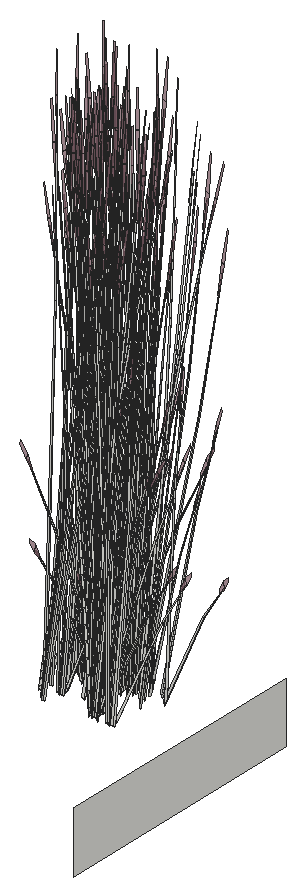
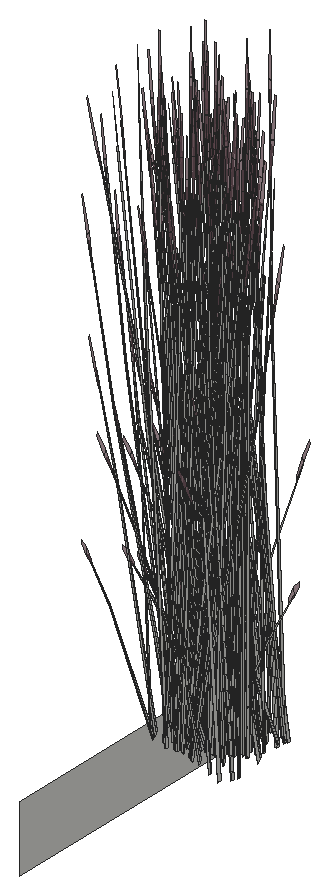
# SketchUp Ruby script. Lengths in inches.
U = 1.inch
M = Sketchup.active_model
def pt(a) = Geom::Point3d.new(a.map { |v| v * U })
def face(e, loops, mat)
  f = e.add_face(loops[0].map { |a| pt(a) })
  loops[1..].each { |l| e.add_face(l.map { |a| pt(a) }).erase! }
  f.material = f.back_material = mat if mat
  f
end
# faces: each face lists its corners as indices into pts; further lists are holes
def faces(e, pts, list, mat = nil) = list.each { |f| face(e, (f[0].is_a?(Array) ? f : [f]).map { |l| l.map { |i| pts[i] } }, mat) }
# xy, xz, yz: faces in a plane at the given z, y or x. An outline is a flat list of corners, or four numbers for a rectangle; further outlines are holes
def ring(l) = l.size == 4 ? [[l[0], l[1]], [l[2], l[1]], [l[2], l[3]], [l[0], l[3]]] : l.each_slice(2).to_a
def flat(e, list, mat, &to3) = list.each { |f| face(e, (f[0].is_a?(Array) ? f : [f]).map { |l| ring(l).map { |u, v| to3.(u, v) } }, mat) }
def xy(e, z, list, mat = nil) = flat(e, list, mat) { |x, y| [x, y, z] }
def xz(e, y, list, mat = nil) = flat(e, list, mat) { |x, z| [x, y, z] }
def yz(e, x, list, mat = nil) = flat(e, list, mat) { |y, z| [x, y, z] }
def lines(e, pts, list) = list.each { |a, b| e.add_line(pt(pts[a]), pt(pts[b])) }
# prism: a flat outline (further loops are holes) pulled along v
def prism(e, loops, v, mat = nil)
  f = face(e, loops, mat); d = Geom::Vector3d.new(v.map { |x| x * U })
  f.pushpull(f.normal.samedirection?(d) ? d.length : -d.length)
end
def box(e, o, s, mat = nil) = prism(e, [[o, [o[0] + s[0], o[1], o[2]], [o[0] + s[0], o[1] + s[1], o[2]], [o[0], o[1] + s[1], o[2]]]], [0, 0, s[2]], mat)
def at(x, y, z, deg = 0) = Geom::Transformation.translation(pt([x, y, z])) * Geom::Transformation.rotation(ORIGIN, Z_AXIS, deg.degrees)
def axes(o, x, y, z) = Geom::Transformation.new([*x, 0, *y, 0, *z, 0, *pt(o).to_a, 1])
def part(name) = M.definitions.add(name)
# library, detail: a bought-in or finely detailed component or shape, given as its bounding box
def library(name, o, s) = part(name).tap { |d| box(d.entities, o, s) }
def detail(e, o, s) = box(e.add_group.entities, o, s)
def put(e, d, t, mat = nil) = e.add_instance(d, t).tap { |i| i.material = mat if mat }
def group(e, t, mat = nil) = e.add_group.tap { |g| g.transformation = t; g.material = mat if mat }.entities
root = M.entities
M.materials.add("LightPink_Translucent").color = [144, 107, 117]
M.materials["LightPink_Translucent"].alpha = 0.75
c1 = part("blade")
p = [[2.15,0.21,22],[0,0.17,0],[0.09,0.45,0],[2.18,0.31,22],[2.29,0.31,22],[0.38,0.45,0],
  [2.48,0.24,33],[2.49,0.24,33],[2.48,0.22,33]]
faces(c1.entities,p,[[0,1,2,3],[4,5,2,3],[6,3,4,7],[8,0,3,6]])
c2 = part("seeds")
p = [[0.3,-0.1,1.38],[-0.01,-0.03,1.59],[-0.01,-0.03,0.03],[0.14,-0.07,-0.07],[0.29,-0.03,3],[0.15,0.01,3.11]]
faces(c2.entities,p,[[0,1,2,3],[1,0,4,5]],"LightPink_Translucent")
c3 = part("blade with seeds")
put(c3.entities,c1,at(0,0,0))
put(c3.entities,c2,axes([2.4,0.25,30.99],[1.5799,-0.05474,1.17369],[-0.12525,1.92788,0.29478],[-0.07173,-0.02425,1.56792]))
yz(root,346,[[14,42,40,48]])
put(root,c3,axes([334.63,24.32,49.95],[0.56491,0,0],[0,0.40454,0],[0,0,1.5764]))
put(root,c3,axes([339.08,29.64,49.82],[-0.52523,-0.06406,-0.55095],[0.11084,-0.39517,-0.1446],[-0.15674,-0.04788,1.21613]))
put(root,c3,axes([336.74,29.35,50.19],[0.47255,-0.19538,0.43871],[0.28245,0.35034,0],[-0.10763,0.0445,1.3917]))
put(root,c3,axes([334.83,24.28,50.3125],[0.47043,-0.11396,0.12794],[0.16474,0.32541,-0.36534],[0,0.07162,1.11991]))
put(root,c3,axes([335.26,27.95,50.09],[0.21952,0.43694,0.40429],[-0.62724,0.15194,0.15865],[0.00767,-0.08029,1.40366]))
put(root,c3,axes([335.16,27.9,49.95],[0.24498,-0.3521,-0.39531],[0.50902,0.16945,0.19025],[0,-0.08116,1.26923]))
put(root,c3,axes([335.79,29.03,49.95],[-0.16474,-0.33688,0],[0.47043,-0.11798,0],[0,0,1.36402]))
put(root,c3,axes([333.85,30.61,50.1],[-0.31568,-0.39156,0],[0.52815,-0.21836,-0.456],[0.12029,-0.04973,1.44655]))
put(root,c3,axes([334.67,24.3,50.36],[0.56863,0.18645,-0.25709],[-0.2738,0.39352,-0.44182],[0.01787,0.09662,1.41118]))
put(root,c3,axes([338.39,30.38,49.78],[-0.47255,-0.19538,-0.43871],[0.28245,-0.35034,0],[-0.10763,-0.0445,1.3917]))
put(root,c3,axes([338.18,27.47,49.32],[-0.04891,0.05148,1.55816],[-0.49427,0.11098,-0.23804],[-0.1194,-0.10096,0.26541]))
put(root,c3,axes([335.9,24.39,50.19],[0,-0.39075,0.43871],[0.56491,0,0],[0,0.089,1.3917]))
put(root,c3,axes([336.15,24.76,49.78],[0,0.39075,-0.43871],[-0.56491,0,0],[0,0.089,1.3917]))
put(root,c3,axes([337.42,28.15,50.1875],[-0.39671,-0.28463,0.15589],[0.39978,-0.27607,0.31002],[-0.04381,0.05813,1.41735]))
put(root,c3,axes([336.05,27.99,49.95],[0,-0.45213,0],[0.63136,0,0],[0,0,1.58567]))
put(root,c3,axes([335.46,28.07,50.15],[0.56891,0.18939,0.21263],[-0.2738,0.39352,0.44182],[0,-0.09071,1.41855]))
put(root,c3,axes([336.37,28.17,50.03],[0,0.45191,-0.04981],[-0.63136,0,0],[0,0.0142,1.58489]))
put(root,c3,axes([335.28,27.81,50.4],[-0.54829,0.02412,0.39531],[-0.04958,-0.40041,-0.19025],[0.09816,-0.04058,1.26923]))
put(root,c3,axes([338.1,24.99,50.29],[0.15933,-0.06164,1.26356],[0.39339,0.18587,-0.27174],[-0.11709,0.16083,0.54024]))
put(root,c3,axes([337.88,27.67,49.88],[-0.14565,0.31907,-0.0344],[-0.44829,-0.09815,-0.15595],[-0.06806,-0.05219,0.51438]))
put(root,c3,axes([335.02,27.12,50.1875],[-0.14586,0.38834,0.15589],[-0.53375,-0.1099,0.31002],[0.0922,-0.00189,1.41735]))
put(root,c3,axes([334.56,25.21,49.93],[0.53009,-0.13258,-0.16963],[0.18627,0.38191,0.00007],[0.05851,-0.01465,1.53656]))
put(root,c3,axes([338.55,27.27,50.29],[-0.03058,0.12783,1.26356],[-0.44698,0.10701,-0.27174],[-0.10448,-0.16522,0.54024]))
put(root,c3,axes([339.68,29.69,50.36],[-0.50979,0.25942,-0.25709],[-0.339,-0.36656,-0.44182],[-0.12578,-0.03723,1.41118]))
put(root,c3,axes([334.76,26.64,50.1],[-0.31568,-0.39156,0],[0.52815,-0.21836,-0.456],[0.12029,-0.04973,1.44655]))
put(root,c3,axes([334.57,24.08,49.95],[0.30332,0.32798,-0.39531],[-0.45944,0.23096,0.19025],[0.09816,0.04058,1.26923]))
put(root,c3,axes([336.64,27.14,50.1875],[-0.54257,0.10371,0.15589],[-0.13397,-0.38597,0.31002],[0.04839,0.05624,1.41735]))
put(root,c3,axes([337.64,29.13,50.1],[-0.63136,0,0],[0,-0.43672,-0.456],[0,-0.09947,1.44655]))
put(root,c3,axes([338.52,30.24,49.79],[-0.11861,-0.34048,-0.27372],[0.47106,-0.09668,0.27372],[-0.09497,-0.03926,1.22797]))
put(root,c3,axes([335.7,30.3,50.29],[-0.14352,0.07909,1.26356],[-0.42983,-0.13843,-0.27174],[0.07968,-0.17216,0.54024]))
put(root,c3,axes([335.75,27.7,50.09],[-0.41865,0.35461,0.40429],[-0.49737,-0.31303,0.15865],[0.10093,-0.03539,1.40366]))
put(root,c3,axes([334.42,25.45,50.29],[0.00891,-0.12953,1.26356],[0.4258,-0.14469,-0.27174],[0.13144,0.15503,0.54024]))
put(root,c3,axes([336.47,28.26,49.96],[0.35245,0.2524,0],[-0.35245,0.2524,0],[0,0,1.49564]))
put(root,c3,axes([336.46,27.97,50.4],[0.24498,-0.3521,0.39531],[0.50902,0.16945,-0.19025],[0,0.08116,1.26923]))
put(root,c3,axes([336.25,29.19,49.95],[0.50902,0.17543,0],[-0.24498,0.36452,0],[0,0,1.54589]))
put(root,c3,axes([340.02,23.79,49.82],[-0.34009,0.2937,-0.55095],[-0.42248,-0.26632,-0.1446],[-0.13628,0.07327,1.21613]))
put(root,c3,axes([334.28,30.55,49.78],[0.47255,-0.19538,-0.43871],[0.28245,0.35034,0],[0.10763,-0.0445,1.3917]))
put(root,c3,axes([338.125,29.01,50.06],[-0.46965,0.32852,0.27176],[-0.46994,-0.32506,-0.32244],[-0.0164,-0.09329,1.45692]))
put(root,c3,axes([336.3,27.88,50.1],[-0.63817,-0.08233,0.43472],[0.12987,-0.46497,0.17059],[0.09326,0.0449,1.50931]))
put(root,c3,axes([335.4,23.35,49.79],[0.11861,0.34048,-0.27372],[-0.47106,0.09668,0.27372],[0.09497,0.03926,1.22797]))
put(root,c3,axes([336.29,24.46,50.1],[0.63136,0,0],[0,0.43672,-0.456],[0,0.09947,1.44655]))
put(root,c3,axes([340.25,29.8125,50.18],[-0.49304,-0.31451,-0.2226],[0.41487,-0.35316,0.48713],[-0.13277,0.03679,1.48635]))
put(root,c3,axes([339.35,29.51,49.95],[-0.30332,-0.32798,-0.39531],[0.45944,-0.23096,0.19025],[-0.09816,-0.04058,1.26923]))
put(root,c3,axes([336.48,28.09,49.95],[0.56491,0,0],[0,0.40454,0],[0,0,1.5764]))
put(root,c3,axes([335.47,26.08,50.36],[-0.32378,-0.01225,0.92831],[0.21383,-0.26028,0.51254],[0.12791,0.09247,0.72818]))
put(root,c3,axes([335.93,27.64,50.4],[-0.30332,-0.32798,0.39531],[0.45944,-0.23096,-0.19025],[0.09816,0.04058,1.26923]))
put(root,c3,axes([335.38,27.72,50.36],[-0.05884,-0.44587,-0.25709],[0.6128,-0.02696,-0.44182],[0.10791,-0.05939,1.41118]))
put(root,c3,axes([336.67,28.05,50.3125],[0.47043,-0.11396,0.12794],[0.16474,0.32541,-0.36534],[0,0.07162,1.11991]))
put(root,c3,axes([338.95,30.42,50.19],[0.47255,0.19538,0.43871],[-0.28245,0.35034,0],[-0.10763,-0.0445,1.3917]))
put(root,c3,axes([335.3,26.74,49.79],[0.47106,0.09668,-0.27372],[-0.11861,0.34048,0.27372],[0.09497,-0.03926,1.22797]))
put(root,c3,axes([339.4,29.7,50.16],[0.13383,-0.46302,-0.20702],[0.63453,0.08071,0.45303],[-0.11087,-0.06394,1.38231]))
put(root,c3,axes([339.63,29.81,50.3125],[-0.09741,0.34873,0.12794],[-0.4759,-0.06053,-0.36534],[-0.08661,-0.03581,1.11991]))
put(root,c3,axes([337.75,28.17,50.19],[0,-0.39075,0.43871],[0.56491,0,0],[0,0.089,1.3917]))
put(root,c3,axes([335.19,26.58,49.78],[0.47255,-0.19538,-0.43871],[0.28245,0.35034,0],[0.10763,-0.0445,1.3917]))
put(root,c3,axes([340.58,24.59,49.78],[-0.47255,0.19538,-0.43871],[-0.28245,-0.35034,0],[-0.10763,0.0445,1.3917]))
put(root,c3,axes([334.84,31.35,49.82],[0.34009,-0.2937,-0.55095],[0.42248,0.26632,-0.1446],[0.13628,-0.07327,1.21613]))
put(root,c3,axes([337.78,28.83,49.78],[0,-0.39075,-0.43871],[0.56491,0,0],[0,-0.089,1.3917]))
put(root,c3,axes([338.02,29.2,50.19],[0,0.39075,0.43871],[-0.56491,0,0],[0,-0.089,1.3917]))
put(root,c3,axes([340.61,24.48,49.9375],[-0.31175,-0.39292,-0.04544],[0.52815,-0.21836,0.456],[-0.13015,0.03741,1.44584]))
put(root,c3,axes([336.14,27.55,50.3125],[0.09741,-0.34873,0.12794],[0.4759,0.06053,-0.36534],[0.08661,0.03581,1.11991]))
put(root,c3,axes([340.46,24.43,49.79],[-0.47106,-0.09668,-0.27372],[0.11861,-0.34048,0.27372],[-0.09497,0.03926,1.22797]))
put(root,c3,axes([335.53,23.2,49.78],[0.47255,0.19538,-0.43871],[-0.28245,0.35034,0],[0.10763,0.0445,1.3917]))
put(root,c3,axes([336.81,26.94,50.19],[-0.47255,-0.19538,0.43871],[0.28245,-0.35034,0],[0.10763,0.0445,1.3917]))
put(root,c3,axes([339.25,29.28,50.36],[-0.56863,-0.18645,-0.25709],[0.2738,-0.39352,-0.44182],[-0.01787,-0.09662,1.41118]))
put(root,c3,axes([335.51,25.98,49.32],[0.03679,-0.05641,1.55816],[0.46313,-0.16615,-0.23804],[0.14041,0.08599,0.26541]))
put(root,c3,axes([336.4,28.99,49.93],[0.53009,-0.13258,-0.16963],[0.18627,0.38191,0.00007],[0.05851,-0.01465,1.53656]))
put(root,c3,axes([338.21,24.7,50.49],[0.45869,-0.0692,0.0575],[0.10545,0.27878,-0.76259],[-0.02908,0.14112,0.68355]))
put(root,c3,axes([340.38,23.44,50.36],[0.05884,0.44587,-0.25709],[-0.6128,0.02696,-0.44182],[-0.10791,0.05939,1.41118]))
put(root,c3,axes([339,28.89,49.85],[-0.20736,-0.4007,-0.61707],[0.59731,-0.14431,-0.16195],[-0.02292,-0.13569,1.36206]))
put(root,c3,axes([334.84,23.95,49.82],[0.52523,0.06406,-0.55095],[-0.11084,0.39517,-0.1446],[0.15674,0.04788,1.21613]))
put(root,c3,axes([336.41,27.85,49.95],[0.30332,0.32798,-0.39531],[-0.45944,0.23096,0.19025],[0.09816,0.04058,1.26923]))
put(root,c3,axes([338.02,28.84,49.79],[0.35245,-0.2438,-0.27372],[0.35245,0.2438,0.27372],[0,-0.07853,1.22797]))
put(root,c3,axes([339.61,27.26,49.88],[-0.34892,0.22417,-0.0344],[-0.3197,-0.24551,-0.15595],[-0.02251,-0.06957,0.51438]))
put(root,c3,axes([339.47,29.48,50.09],[0.63817,0.08233,0.40429],[-0.12987,0.46497,0.15865],[-0.09326,-0.0449,1.40366]))
put(root,c3,axes([335.75,27.38,49.82],[0.34009,-0.2937,-0.55095],[0.42248,0.26632,-0.1446],[0.13628,-0.07327,1.21613]))
put(root,c3,axes([339.31,29.39,50.4],[-0.24498,0.3521,0.39531],[-0.50902,-0.16945,-0.19025],[0,-0.08116,1.26923]))
put(root,c3,axes([336.71,30.54,49.32],[-0.07557,-0.03078,1.55816],[-0.19412,-0.34391,-0.23804],[0.13095,-0.09333,0.26541]))
put(root,c3,axes([337.24,27.12,49.79],[0.11861,0.34048,-0.27372],[-0.47106,0.09668,0.27372],[0.09497,0.03926,1.22797]))
put(root,c3,axes([339.13,30.22,50.1875],[0.54257,-0.10371,0.15589],[0.13397,0.38597,0.31002],[-0.04839,-0.05624,1.41735]))
put(root,c3,axes([339.83,30.28,49.94],[-0.50902,-0.17543,0],[0.24498,-0.36452,0],[0,0,1.43768]))
put(root,c3,axes([341,24.53,50.1],[0.31568,0.39156,0],[-0.52815,0.21836,-0.456],[-0.12029,0.04973,1.44655]))
put(root,c3,axes([336.09,27.67,50.36],[0.50979,-0.25942,-0.25709],[0.339,0.36656,-0.44182],[0.12578,0.03723,1.41118]))
put(root,c3,axes([340.74,30.24,50.1875],[0.14586,-0.38834,0.15589],[0.53375,0.1099,0.31002],[-0.0922,0.00189,1.41735]))
put(root,c3,axes([340.5,23.53,50.3125],[0.37303,0.23477,0.12794],[-0.31115,0.26487,-0.36534],[-0.08661,0.03581,1.11991]))
put(root,c3,axes([340.36,29.43,50.03],[-0.46965,-0.33633,-0.05417],[0.46994,-0.33653,0],[-0.0164,-0.01174,1.55135]))
put(root,c3,axes([334.8,27.43,49.41],[-0.49699,0.15644,1.13921],[-0.15819,-0.44887,0.44265],[0.30518,0.00747,1.29573]))
put(root,c3,axes([340.62,24.28,50.06],[0.63212,0.12701,0.27176],[-0.15814,0.45398,-0.32244],[-0.10462,0.05682,1.45692]))
put(root,c3,axes([339.7,26.99,49.32],[-0.08469,0.01408,1.55816],[-0.46834,-0.15847,-0.23804],[0.00786,-0.13218,0.26541]))
put(root,c3,axes([340.89,24.26,50.19],[0.47255,-0.19538,0.43871],[0.28245,0.35034,0],[-0.10763,0.0445,1.3917]))
put(root,c3,axes([339.42,29.05,50.09],[0.21952,0.43694,0.40429],[-0.62724,0.15194,0.15865],[0.00767,-0.08029,1.40366]))
put(root,c3,axes([339.32,28.99,49.95],[0.24498,-0.3521,-0.39531],[0.50902,0.16945,0.19025],[0,-0.08116,1.26923]))
put(root,c3,axes([339.94,30.13,49.95],[-0.16474,-0.33688,0],[0.47043,-0.11798,0],[0,0,1.36402]))
put(root,c3,axes([339.34,24.65,49.32],[0.08172,-0.02126,1.55816],[0.49154,0.11703,-0.23804],[0.01437,0.1319,0.26541]))
put(root,c3,axes([337.09,26.74,50.1],[0.31568,-0.39156,0],[0.52815,0.21836,-0.456],[0.12029,0.04973,1.44655]))
put(root,c3,axes([337.62,26.57,49.32],[-0.07557,-0.03078,1.55816],[-0.19412,-0.34391,-0.23804],[0.13095,-0.09333,0.26541]))
put(root,c3,axes([337.375,26.98,49.78],[0.47255,0.19538,-0.43871],[-0.28245,0.35034,0],[0.10763,0.0445,1.3917]))
put(root,c3,axes([340.61,23.27,49.95],[-0.24498,0.3521,-0.39531],[-0.50902,-0.16945,0.19025],[0,0.08116,1.26923]))
put(root,c3,axes([336.6875,27.72,49.82],[0.52523,0.06406,-0.55095],[-0.11084,0.39517,-0.1446],[0.15674,0.04788,1.21613]))
put(root,c3,axes([341.58,29.25,50.1875],[-0.39671,-0.28463,0.15589],[0.39978,-0.27607,0.31002],[-0.04381,0.05813,1.41735]))
put(root,c3,axes([338.92,27.96,50],[-0.31304,-0.24986,-0.05733],[0.34284,-0.22894,-0.25992],[0.09714,-0.01612,0.85731]))
put(root,c3,axes([340.21,29.08,49.95],[0,-0.45213,0],[0.63136,0,0],[0,0,1.58567]))
put(root,c3,axes([339.62,29.17,50.15],[0.56891,0.18939,0.21263],[-0.2738,0.39352,0.44182],[0,-0.09071,1.41855]))
put(root,c3,axes([339.44,28.9,50.4],[-0.54829,0.02412,0.39531],[-0.04958,-0.40041,-0.19025],[0.09816,-0.04058,1.26923]))
put(root,c3,axes([339.18,28.22,50.1875],[-0.14586,0.38834,0.15589],[-0.53375,-0.1099,0.31002],[0.0922,-0.00189,1.41735]))
put(root,c3,axes([340.22,23.95,50.02],[0.21952,0.44891,-0.05313],[-0.62724,0.1573,0],[0.00767,0.01568,1.52132]))
put(root,c3,axes([338.92,27.74,50.1],[-0.31568,-0.39156,0],[0.52815,-0.21836,-0.456],[0.12029,-0.04973,1.44655]))
put(root,c3,axes([342.03,23.36,49.94],[-0.63105,-0.00312,-0.04397],[0,-0.43672,0.44129],[-0.01983,0.09942,1.3992]))
put(root,c3,axes([337.09,31.23,50.29],[-0.18038,-0.01157,1.26356],[-0.18479,-0.31048,-0.27174],[0.22159,-0.08783,0.54024]))
put(root,c3,axes([340.79,28.24,50.1875],[-0.54257,0.10371,0.15589],[-0.13397,-0.38597,0.31002],[0.04839,0.05624,1.41735]))
put(root,c3,axes([336.58,25.07,50.29],[-0.1216,-0.0961,1.26356],[0.15822,-0.31792,-0.27174],[0.24603,0.04307,0.54024]))
put(root,c3,axes([339.91,28.8,50.09],[-0.41865,0.35461,0.40429],[-0.49737,-0.31303,0.15865],[0.10093,-0.03539,1.40366]))
put(root,c3,axes([340.62,29.36,49.96],[0.35245,0.2524,0],[-0.35245,0.2524,0],[0,0,1.49564]))
put(root,c3,axes([340.4,24.09,49.95],[0.50902,0.17543,0],[-0.24498,0.36452,0],[0,0,1.54589]))
put(root,c3,axes([340.45,28.98,50.1],[-0.63817,-0.08233,0.43472],[0.12987,-0.46497,0.17059],[0.09326,0.0449,1.50931]))
put(root,c3,axes([341.9,23.42,49.79],[-0.35245,0.2438,-0.27372],[-0.35245,-0.2438,0.27372],[0,0.07853,1.22797]))
put(root,c3,axes([340.9,23.375,49.85],[0.18514,0.35777,-0.61156],[-0.53331,0.12885,-0.16051],[0.02046,0.12115,1.3499]))
put(root,c3,axes([340.63,29.19,49.95],[0.56491,0,0],[0,0.40454,0],[0,0,1.5764]))
put(root,c3,axes([340.09,28.74,50.4],[-0.30332,-0.32798,0.39531],[0.45944,-0.23096,-0.19025],[0.09816,0.04058,1.26923]))
put(root,c3,axes([339.54,28.82,50.36],[-0.05884,-0.44587,-0.25709],[0.6128,-0.02696,-0.44182],[0.10791,-0.05939,1.41118]))
put(root,c3,axes([338,27.26,50.29],[-0.18038,-0.01157,1.26356],[-0.18479,-0.31048,-0.27174],[0.22159,-0.08783,0.54024]))
put(root,c3,axes([340.67,22.98,50.36],[0.56863,0.18645,-0.25709],[-0.2738,0.39352,-0.44182],[0.01787,0.09662,1.41118]))
put(root,c3,axes([339.46,27.83,49.79],[0.47106,0.09668,-0.27372],[-0.11861,0.34048,0.27372],[0.09497,-0.03926,1.22797]))
put(root,c3,axes([340.77,27.42,50.29],[-0.14352,0.07909,1.26356],[-0.42983,-0.13843,-0.27174],[0.07968,-0.17216,0.54024]))
put(root,c3,axes([338.33,28.29,49.75],[-0.3252,0.04689,1.25103],[-0.05176,-0.37326,0.07161],[0.22777,-0.0565,0.71188]))
put(root,c3,axes([338.68,28.04,49.32],[-0.02639,-0.05932,1.55816],[0.18302,-0.34702,-0.23804],[0.18462,-0.00499,0.26541]))
put(root,c3,axes([342.15,23.43,49.78],[0,0.39075,-0.43871],[-0.56491,0,0],[0,0.089,1.3917]))
put(root,c3,axes([339.35,27.68,49.78],[0.47255,-0.19538,-0.43871],[0.28245,0.35034,0],[0.10763,-0.0445,1.3917]))
put(root,c3,axes([340.29,28.65,50.3125],[0.09741,-0.34873,0.12794],[0.4759,0.06053,-0.36534],[0.08661,0.03581,1.11991]))
put(root,c3,axes([340.97,28.04,50.19],[-0.47255,-0.19538,0.43871],[0.28245,-0.35034,0],[0.10763,0.0445,1.3917]))
put(root,c3,axes([340.56,30.08,49.93],[0.53009,-0.13258,-0.16963],[0.18627,0.38191,0.00007],[0.05851,-0.01465,1.53656]))
put(root,c3,axes([338.42,28.84,50.29],[-0.1216,-0.0961,1.26356],[0.15822,-0.31792,-0.27174],[0.24603,0.04307,0.54024]))
put(root,c3,axes([340.42,24.12,50.29],[0.00891,-0.12953,1.26356],[0.4258,-0.14469,-0.27174],[0.13144,0.15503,0.54024]))
put(root,c3,axes([339.91,28.48,49.82],[0.34009,-0.2937,-0.55095],[0.42248,0.26632,-0.1446],[0.13628,-0.07327,1.21613]))
put(root,c3,axes([341.4,28.22,49.79],[0.11861,0.34048,-0.27372],[-0.47106,0.09668,0.27372],[0.09497,0.03926,1.22797]))
put(root,c3,axes([342.29,23.13,50.1],[0.63136,0,0],[0,0.43672,-0.456],[0,0.09947,1.44655]))
put(root,c3,axes([340.25,28.76,50.36],[0.50979,-0.25942,-0.25709],[0.339,0.36656,-0.44182],[0.12578,0.03723,1.41118]))
put(root,c3,axes([341.47,24.75,50.36],[-0.32378,-0.01225,0.92831],[0.21383,-0.26028,0.51254],[0.12791,0.09247,0.72818]))
put(root,c3,axes([338.96,28.53,49.41],[-0.49699,0.15644,1.13921],[-0.15819,-0.44887,0.44265],[0.30518,0.00747,1.29573]))
put(root,c3,axes([341.24,27.83,50.1],[0.31568,-0.39156,0],[0.52815,0.21836,-0.456],[0.12029,0.04973,1.44655]))
put(root,c3,axes([341.77,27.66,49.32],[-0.07557,-0.03078,1.55816],[-0.19412,-0.34391,-0.23804],[0.13095,-0.09333,0.26541]))
put(root,c3,axes([341.53,28.07,49.78],[0.47255,0.19538,-0.43871],[-0.28245,0.35034,0],[0.10763,0.0445,1.3917]))
put(root,c3,axes([341.51,24.66,49.32],[0.03679,-0.05641,1.55816],[0.46313,-0.16615,-0.23804],[0.14041,0.08599,0.26541]))
put(root,c3,axes([340.84,28.82,49.82],[0.52523,0.06406,-0.55095],[-0.11084,0.39517,-0.1446],[0.15674,0.04788,1.21613]))
put(root,c3,axes([343.08,29.05,50],[-0.31304,-0.24986,-0.05733],[0.34284,-0.22894,-0.25992],[0.09714,-0.01612,0.85731]))
put(root,c3,axes([342.15,28.35,50.29],[-0.18038,-0.01157,1.26356],[-0.18479,-0.31048,-0.27174],[0.22159,-0.08783,0.54024]))
put(root,c3,axes([342.49,29.38,49.75],[-0.3252,0.04689,1.25103],[-0.05176,-0.37326,0.07161],[0.22777,-0.0565,0.71188]))
put(root,c3,axes([342.84,29.14,49.32],[-0.02639,-0.05932,1.55816],[0.18302,-0.34702,-0.23804],[0.18462,-0.00499,0.26541]))
